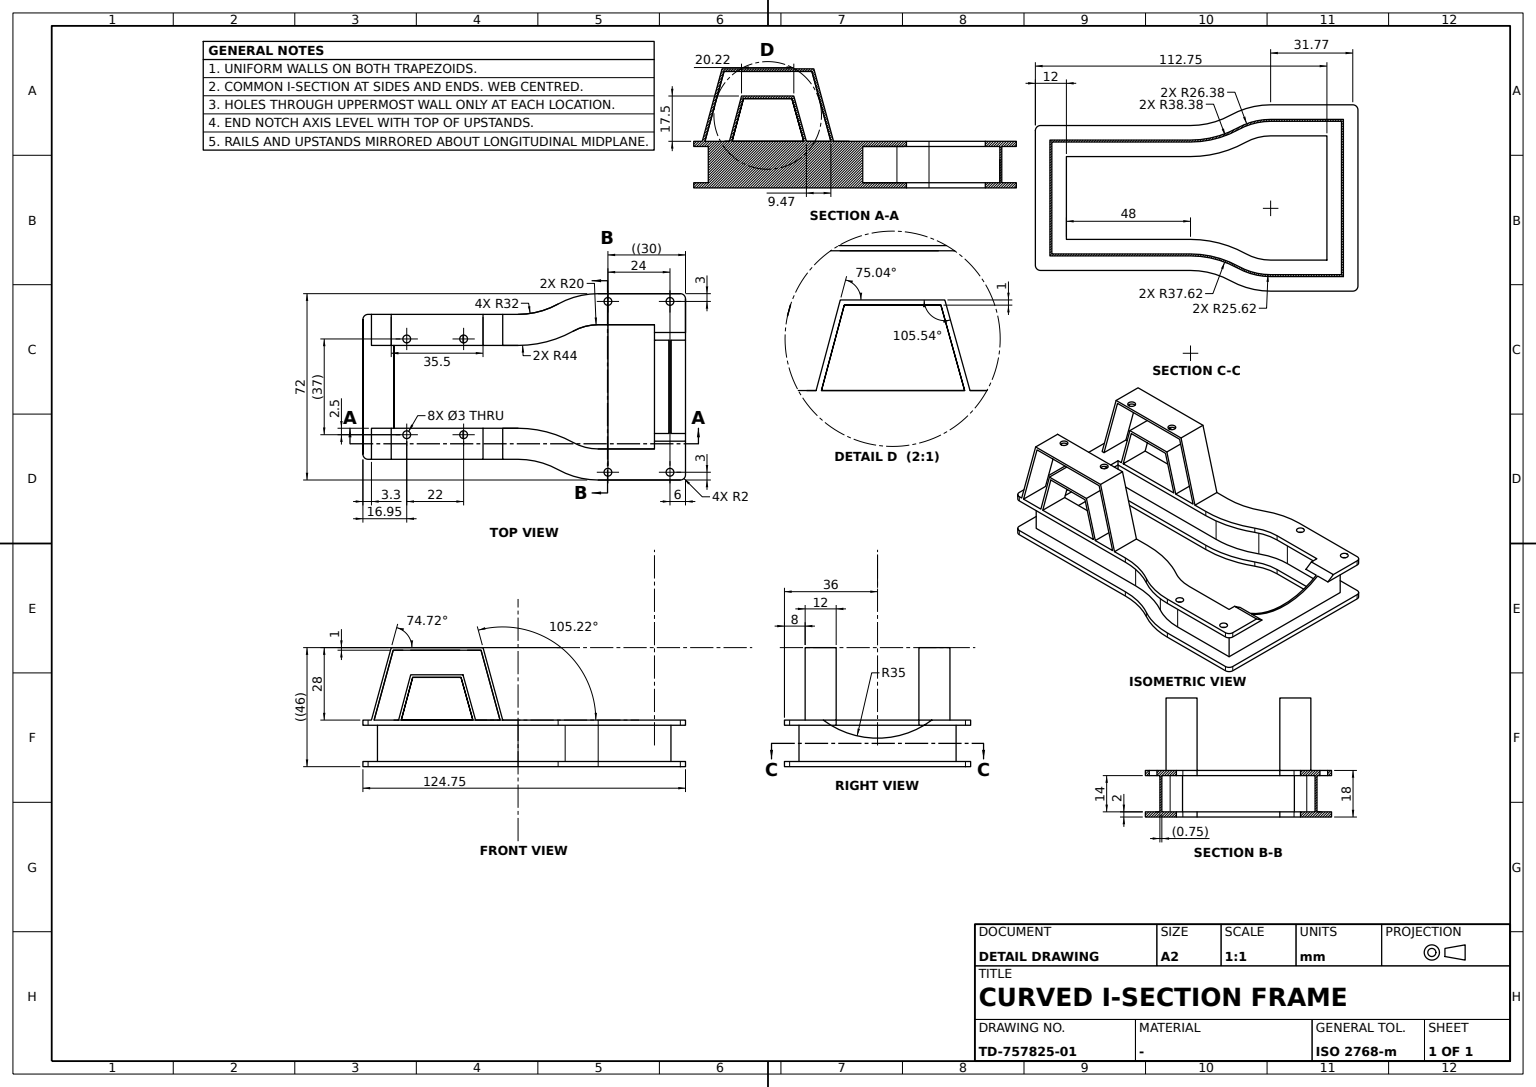
solid
v1 (-27.078125,72.215125,7)
v2 (-30.375,84.983867,7)
e1 v1 v2 CIRCLE(AX(P(-4,84.983867,7),D(0,0,1),D(1,0,0)),26.375) rev
v3 (-30.375,84.983867,-7)
e2 v3 v2 LINE
v4 (-27.078125,72.215125,-7)
e3 v4 v3 CIRCLE(AX(P(-4,84.983867,-7),D(0,0,-1),D(-1,0,0)),26.375)
e4 v4 v1 LINE
face CYL(AX(P(-4,84.983867,0),D(0,0,-1),D(-0.875,-0.484122918,0)),26.375) [e1 -e2 -e3 e4]
v5 (-16,47.031009,9)
v6 (-16,37.565009,9)
e5 v5 v6 LINE
v7 (-28,47.031009,9)
e6 v7 v5 LINE
v8 (-28,37.565009,9)
e7 v8 v7 LINE
e8 v8 v6 LINE
face PLANE(AX(P(0,-6,9),D(0,0,-1),D(0,1,0))) rev [-e5 -e6 -e7 e8]
v9 (-28,36.527057,9)
v10 (-16,36.527057,9)
e9 v9 v10 LINE
v11 (-28,8.837722,9)
e10 v11 v9 LINE
v12 (-16,8.837722,9)
e11 v11 v12 LINE
e12 v10 v12 LINE
face PLANE(AX(P(0,-6,9),D(0,0,-1),D(0,1,0))) rev [-e9 -e10 e11 -e12]
v13 (-32,69.491933,-9)
v14 (-36,84.983867,-9)
e13 v13 v14 CIRCLE(AX(P(-4,84.983867,-9),D(0,0,1),D(1,0,0)),32) rev
v15 (-32,69.491933,-7)
e14 v13 v15 LINE
v16 (-36,84.983867,-7)
e15 v15 v16 CIRCLE(AX(P(-4,84.983867,-7),D(0,0,-1),D(-1,0,0)),32)
e16 v14 v16 LINE
face CYL(AX(P(-4,84.983867,0),D(0,0,-1),D(-0.875,-0.484122918,0)),32) [-e13 e14 e15 -e16]
v17 (20,32.949611,36)
e17 v17 v17 CIRCLE(AX(P(18.5,32.949611,36),D(0,0,1),D(1,0,0)),1.5)
v18 (20,32.949611,37)
e18 v18 v18 CIRCLE(AX(P(18.5,32.949611,37),D(0,0,1),D(1,0,0)),1.5)
face CYL(AX(P(18.5,32.949611,13.34),D(0,0,1),D(0,1,0)),1.5) rev [-e17] [e18]
v19 (-16,32.698119,26.5)
e19 v19 v6 LINE
v20 (-28,32.698119,26.5)
e20 v20 v8 LINE
e21 v20 v19 LINE
face PLANE(AX(P(28,32.698119,26.5),D(0,0.963435821,0.267939209),D(0,0.267939209,-0.963435821))) [e19 -e8 -e20 e21]
v21 (24,106.75,-7)
v22 (-24,106.75,-7)
e22 v21 v22 LINE
v23 (-24,106.75,-9)
e23 v23 v22 LINE
v24 (24,106.75,-9)
e24 v24 v23 LINE
e25 v24 v21 LINE
face PLANE(AX(P(42,106.75,-7),D(0,1,0),D(0,0,-1))) rev [e22 -e23 -e24 e25]
v25 (16,13.246024,25.5)
v26 (16,31.938275,25.5)
e26 v25 v26 LINE
v27 (16,8.837722,9)
e27 v27 v25 LINE
v28 (16,36.527057,9)
e28 v28 v27 LINE
e29 v26 v28 LINE
v29 (16,32.698119,26.5)
v30 (16,37.565009,9)
e30 v29 v30 LINE
v31 (16,47.031009,9)
e31 v31 v30 LINE
v32 (16,39.685325,36)
e32 v32 v31 LINE
v33 (16,5.713058,36)
e33 v33 v32 LINE
v34 (16,-1.663352,9)
e34 v34 v33 LINE
v35 (16,-2.7,9)
e35 v35 v34 LINE
v36 (16,4.949611,37)
e36 v35 v36 LINE
v37 (16,40.449611,37)
e37 v36 v37 LINE
v38 (16,48.067357,9)
e38 v37 v38 LINE
v39 (16,54,9)
e39 v39 v38 LINE
v40 (16,54,7)
e40 v39 v40 LINE
v41 (16,6,7)
e41 v41 v40 LINE
v42 (16,6,9)
e42 v41 v42 LINE
v43 (16,7.802648,9)
e43 v43 v42 LINE
v44 (16,12.478119,26.5)
e44 v43 v44 LINE
e45 v44 v29 LINE
face PLANE(AX(P(16,-12,-7),D(1,0,0),D(0,0,-1))) rev [-e26 -e27 -e28 -e29] [e30 -e31 -e32 -e33 -e34 -e35 e36 e37 e38 -e39 e40 -e41 e42 -e43 e44 e45]
v45 (24,84.983867,-7)
v46 (24,84.983867,-9)
e46 v45 v46 LINE
e47 v45 v21 LINE
e48 v46 v24 LINE
face PLANE(AX(P(24,84.983867,-7),D(1,0,0),D(0,0,-1))) rev [-e46 e47 -e25 -e48]
v47 (28,-1.663352,9)
e49 v47 v34 LINE
v48 (28,5.713058,36)
e50 v48 v33 LINE
e51 v47 v48 LINE
face PLANE(AX(P(28,-1.663352,9),D(0,-0.964647876,0.263542168),D(0,0.263542168,0.964647876))) rev [e49 e34 -e50 -e51]
v49 (24,84.983867,9)
v50 (24,84.983867,7)
e52 v49 v50 LINE
v51 (21.5,75.301408,7)
e53 v51 v50 CIRCLE(AX(P(4,84.983867,7),D(0,0,1),D(1,0,0)),20)
v52 (21.5,75.301408,9)
e54 v52 v51 LINE
e55 v52 v49 CIRCLE(AX(P(4,84.983867,9),D(0,0,-1),D(-1,0,0)),20) rev
face CYL(AX(P(4,84.983867,0),D(0,0,1),D(0.875,-0.484122918,0)),20) rev [e52 -e53 -e54 e55]
v53 (-29.625,84.983867,7)
v54 (-29.625,112.375,7)
e56 v53 v54 LINE
v55 (-29.625,84.983867,-7)
e57 v53 v55 LINE
v56 (-29.625,112.375,-7)
e58 v55 v56 LINE
e59 v56 v54 LINE
face PLANE(AX(P(-29.625,84.983867,7),D(1,0,0),D(0,0,-1))) [-e56 e57 e58 e59]
v57 (22.375,54,-7)
v58 (22.375,54,7)
e60 v57 v58 LINE
v59 (22.375,-0.375,7)
e61 v59 v58 LINE
v60 (22.375,-0.375,-7)
e62 v59 v60 LINE
e63 v60 v57 LINE
face PLANE(AX(P(22.375,-12,-7),D(-1,0,0),D(0,0,1))) rev [e60 -e61 e62 e63]
v61 (31.5,88.75,9)
e64 v61 v61 CIRCLE(AX(P(33,88.75,9),D(0,0,-1),D(-1,0,0)),1.5) rev
v62 (34.5,88.75,7)
e65 v62 v62 CIRCLE(AX(P(33,88.75,7),D(0,0,1),D(1,0,0)),1.5)
face CYL(AX(P(33,88.75,-0.66),D(0,0,1),D(0,1,0)),1.5) rev [e64] [-e65]
v63 (-28,12.478119,26.5)
e66 v63 v20 LINE
v64 (-16,12.478119,26.5)
e67 v63 v64 LINE
e68 v64 v19 LINE
face PLANE(AX(P(28,12.478119,26.5),D(0,0,1),D(0,1,0))) [-e66 e67 e68 -e21]
v65 (32,69.491933,7)
v66 (32,69.491933,9)
e69 v65 v66 LINE
v67 (36,84.983867,7)
e70 v65 v67 CIRCLE(AX(P(4,84.983867,7),D(0,0,1),D(1,0,0)),32)
v68 (36,84.983867,9)
e71 v67 v68 LINE
e72 v66 v68 CIRCLE(AX(P(4,84.983867,9),D(0,0,-1),D(-1,0,0)),32) rev
face CYL(AX(P(4,84.983867,0),D(0,0,1),D(0.875,-0.484122918,0)),32) [-e69 e70 e71 -e72]
v69 (-26,-6,7)
v70 (26,-6,7)
e73 v69 v70 LINE
v71 (26,-6,9)
e74 v70 v71 LINE
v72 (-26,-6,9)
e75 v72 v71 LINE
e76 v69 v72 LINE
face PLANE(AX(P(0,-6,-9),D(0,1,0),D(0,0,1))) rev [e73 e74 -e75 -e76]
v73 (28,-4,7)
v74 (28,-4,9)
e77 v73 v74 LINE
e78 v74 v71 CIRCLE(AX(P(26,-4,9),D(0,0,-1),D(-1,0,0)),2)
e79 v70 v73 CIRCLE(AX(P(26,-4,7),D(0,0,1),D(1,0,0)),2)
face CYL(AX(P(26,-4,22),D(0,0,1),D(1,0,0)),2) [e77 e78 -e74 e79]
v75 (-16,6,-9)
v76 (-16,54,-9)
e80 v75 v76 LINE
v77 (-16,54,-7)
e81 v77 v76 LINE
v78 (-16,6,-7)
e82 v78 v77 LINE
e83 v75 v78 LINE
face PLANE(AX(P(-16,-12,-7),D(1,0,0),D(0,0,-1))) [e80 -e81 -e82 -e83]
v79 (34,118.75,7)
v80 (34,118.75,9)
e84 v79 v80 LINE
v81 (18.027756,118.75,7)
e85 v79 v81 LINE
v82 (21,118.75,9)
e86 v81 v82 CIRCLE(AX(P(0,118.75,37),D(0,-1,0),D(0,0,-1)),35)
e87 v80 v82 LINE
face PLANE(AX(P(42,118.75,-9),D(0,-1,0),D(0,0,1))) rev [-e84 e85 e86 -e87]
v83 (-31.5,88.75,7)
e88 v83 v83 CIRCLE(AX(P(-33,88.75,7),D(0,0,1),D(1,0,0)),1.5)
v84 (-34.5,88.75,9)
e89 v84 v84 CIRCLE(AX(P(-33,88.75,9),D(0,0,-1),D(-1,0,0)),1.5) rev
face CYL(AX(P(-33,88.75,-0.66),D(0,0,1),D(0,1,0)),1.5) rev [-e88] [e89]
v85 (-28,-2.7,9)
v86 (-16,-2.7,9)
e90 v85 v86 LINE
v87 (-16,4.949611,37)
e91 v86 v87 LINE
v88 (-28,4.949611,37)
e92 v88 v87 LINE
e93 v85 v88 LINE
face PLANE(AX(P(28,-2.7,9),D(0,-0.964647876,0.263542168),D(0,0.263542168,0.964647876))) [e90 e91 -e92 -e93]
v89 (36,116.75,9)
e94 v68 v89 LINE
v90 (36,116.75,7)
e95 v67 v90 LINE
e96 v90 v89 LINE
face PLANE(AX(P(36,84.983867,-9),D(-1,0,0),D(0,0,1))) rev [-e94 -e71 e95 e96]
v91 (-28,-4,7)
e97 v91 v69 CIRCLE(AX(P(-26,-4,7),D(0,0,1),D(1,0,0)),2)
v92 (-28,-4,9)
e98 v72 v92 CIRCLE(AX(P(-26,-4,9),D(0,0,-1),D(-1,0,0)),2)
e99 v91 v92 LINE
face CYL(AX(P(-26,-4,22),D(0,0,1),D(0,-1,0)),2) [e97 e76 e98 -e99]
v93 (28,4.949611,37)
e100 v93 v36 LINE
v94 (28,40.449611,37)
e101 v93 v94 LINE
e102 v94 v37 LINE
v95 (20,10.949611,37)
e103 v95 v95 CIRCLE(AX(P(18.5,10.949611,37),D(0,0,1),D(1,0,0)),1.5)
face PLANE(AX(P(28,4.949611,37),D(0,0,1),D(0,1,0))) [-e18] [-e37 -e100 e101 e102] [-e103]
v96 (18.027756,113.125,7)
e104 v96 v81 LINE
v97 (-18.027756,113.125,7)
e105 v97 v96 CIRCLE(AX(P(0,113.125,37),D(0,-1,0),D(0,0,-1)),35)
v98 (-18.027756,118.75,7)
e106 v98 v97 LINE
v99 (-21,118.75,9)
e107 v99 v98 CIRCLE(AX(P(0,118.75,37),D(0,-1,0),D(0,0,-1)),35)
v100 (-21,106.75,9)
e108 v100 v99 LINE
v101 (-18.027756,106.75,7)
e109 v101 v100 CIRCLE(AX(P(0,106.75,37),D(0,1,0),D(0,0,1)),35)
v102 (-18.027756,112.375,7)
e110 v102 v101 LINE
v103 (18.027756,112.375,7)
e111 v103 v102 CIRCLE(AX(P(0,112.375,37),D(0,1,0),D(0,0,1)),35)
v104 (18.027756,106.75,7)
e112 v104 v103 LINE
v105 (21,106.75,9)
e113 v105 v104 CIRCLE(AX(P(0,106.75,37),D(0,1,0),D(0,0,1)),35)
e114 v82 v105 LINE
face CYL(AX(P(0,115.75,37),D(0,1,0),D(-1,0,0)),35) rev [-e104 -e105 -e106 -e107 -e108 -e109 -e110 -e111 -e112 -e113 -e114 -e86]
v106 (-17,10.949611,36)
e115 v106 v106 CIRCLE(AX(P(-18.5,10.949611,36),D(0,0,1),D(1,0,0)),1.5)
v107 (-17,10.949611,37)
e116 v107 v107 CIRCLE(AX(P(-18.5,10.949611,37),D(0,0,1),D(1,0,0)),1.5)
face CYL(AX(P(-18.5,10.949611,13.34),D(0,0,1),D(0,1,0)),1.5) rev [-e115] [e116]
v108 (-28,54,7)
e117 v91 v108 LINE
v109 (-32,69.491933,7)
e118 v109 v108 CIRCLE(AX(P(-60,54,7),D(0,0,1),D(1,0,0)),32) rev
v110 (-36,84.983867,7)
e119 v109 v110 CIRCLE(AX(P(-4,84.983867,7),D(0,0,1),D(1,0,0)),32) rev
v111 (-36,116.75,7)
e120 v110 v111 LINE
v112 (-34,118.75,7)
e121 v112 v111 CIRCLE(AX(P(-34,116.75,7),D(0,0,1),D(1,0,0)),2)
e122 v98 v112 LINE
v113 (-30.375,113.125,7)
e123 v97 v113 LINE
e124 v2 v113 LINE
v114 (-22.375,54,7)
e125 v1 v114 CIRCLE(AX(P(-60,54,7),D(0,0,1),D(1,0,0)),37.625) rev
v115 (-22.375,-0.375,7)
e126 v115 v114 LINE
e127 v115 v59 LINE
v116 (27.078125,72.215125,7)
e128 v116 v58 CIRCLE(AX(P(60,54,7),D(0,0,1),D(1,0,0)),37.625)
v117 (30.375,84.983867,7)
e129 v116 v117 CIRCLE(AX(P(4,84.983867,7),D(0,0,1),D(1,0,0)),26.375)
v118 (30.375,113.125,7)
e130 v117 v118 LINE
e131 v118 v96 LINE
e132 v90 v79 CIRCLE(AX(P(34,116.75,7),D(0,0,1),D(1,0,0)),2)
v119 (28,54,7)
e133 v65 v119 CIRCLE(AX(P(60,54,7),D(0,0,1),D(1,0,0)),32)
e134 v73 v119 LINE
v120 (-31.5,112.75,7)
e135 v120 v120 CIRCLE(AX(P(-33,112.75,7),D(0,0,1),D(1,0,0)),1.5)
v121 (34.5,112.75,7)
e136 v121 v121 CIRCLE(AX(P(33,112.75,7),D(0,0,1),D(1,0,0)),1.5)
face PLANE(AX(P(0,6,7),D(0,0,1),D(0,-1,0))) rev [e88] [-e97 e117 -e118 e119 e120 -e121 -e122 e106 e123 -e124 -e1 e125 -e126 e127 e61 -e128 e129 e130 e131 e104 -e85 -e132 -e95 -e70 e133 -e134 -e79 -e73] [e65] [e135] [e136]
v122 (16,54,-7)
v123 (16,54,-9)
e137 v122 v123 LINE
v124 (21.5,75.301408,-7)
e138 v124 v122 CIRCLE(AX(P(60,54,-7),D(0,0,-1),D(-1,0,0)),44) rev
v125 (21.5,75.301408,-9)
e139 v124 v125 LINE
e140 v125 v123 CIRCLE(AX(P(60,54,-9),D(0,0,1),D(1,0,0)),44)
face CYL(AX(P(60,54,0),D(0,0,1),D(-0.875,0.484122918,0)),44) [-e137 -e138 e139 e140]
e141 v125 v46 CIRCLE(AX(P(4,84.983867,-9),D(0,0,1),D(1,0,0)),20)
e142 v124 v45 CIRCLE(AX(P(4,84.983867,-7),D(0,0,-1),D(-1,0,0)),20) rev
face CYL(AX(P(4,84.983867,0),D(0,0,1),D(0.875,-0.484122918,0)),20) rev [e46 -e141 -e139 e142]
v126 (-21.5,75.301408,-7)
v127 (-24,84.983867,-7)
e143 v126 v127 CIRCLE(AX(P(-4,84.983867,-7),D(0,0,-1),D(-1,0,0)),20)
v128 (-21.5,75.301408,-9)
e144 v126 v128 LINE
v129 (-24,84.983867,-9)
e145 v128 v129 CIRCLE(AX(P(-4,84.983867,-9),D(0,0,1),D(1,0,0)),20) rev
e146 v127 v129 LINE
face CYL(AX(P(-4,84.983867,0),D(0,0,-1),D(-0.875,-0.484122918,0)),20) rev [-e143 e144 e145 -e146]
v130 (28,7.802648,9)
e147 v130 v43 LINE
v131 (28,12.478119,26.5)
e148 v130 v131 LINE
e149 v131 v44 LINE
face PLANE(AX(P(28,7.802648,9),D(0,-0.966113825,0.258116404),D(0,0.258116404,0.966113825))) [-e147 e148 e149 -e44]
v132 (28,8.837722,9)
e150 v132 v27 LINE
v133 (28,13.246024,25.5)
e151 v133 v25 LINE
e152 v132 v133 LINE
face PLANE(AX(P(28,8.837722,9),D(0,-0.966113825,0.258116404),D(0,0.258116404,0.966113825))) rev [e150 e27 -e151 -e152]
v134 (-28,39.685325,36)
e153 v134 v7 LINE
v135 (-16,39.685325,36)
e154 v135 v5 LINE
e155 v134 v135 LINE
face PLANE(AX(P(28,39.685325,36),D(0,0.964926501,0.262520187),D(0,0.262520187,-0.964926501))) rev [e153 e6 -e154 -e155]
v136 (-22.375,-0.375,-7)
v137 (-22.375,54,-7)
e156 v136 v137 LINE
e157 v115 v136 LINE
e158 v137 v114 LINE
face PLANE(AX(P(-22.375,-12,-7),D(-1,0,0),D(0,0,1))) [-e156 -e157 e126 -e158]
v138 (-16,6,7)
e159 v138 v41 LINE
v139 (-16,6,9)
e160 v138 v139 LINE
e161 v139 v42 LINE
face PLANE(AX(P(0,6,-7),D(0,-1,0),D(0,0,-1))) rev [-e159 e160 e161 -e42]
v140 (21.625,54,7)
v141 (21.625,54,-7)
e162 v140 v141 LINE
v142 (26.421875,72.578217,7)
e163 v142 v140 CIRCLE(AX(P(60,54,7),D(0,0,1),D(1,0,0)),38.375)
v143 (26.421875,72.578217,-7)
e164 v142 v143 LINE
e165 v143 v141 CIRCLE(AX(P(60,54,-7),D(0,0,-1),D(-1,0,0)),38.375) rev
face CYL(AX(P(60,54,0),D(0,0,1),D(-0.875,0.484122918,0)),38.375) [-e162 -e163 e164 e165]
v144 (20,10.949611,36)
e166 v144 v144 CIRCLE(AX(P(18.5,10.949611,36),D(0,0,1),D(1,0,0)),1.5)
v145 (28,39.685325,36)
e167 v145 v32 LINE
e168 v48 v145 LINE
face PLANE(AX(P(28,5.713058,36),D(0,0,1),D(0,1,0))) rev [e17] [e166] [e50 e33 -e167 -e168]
v146 (-32,69.491933,9)
e169 v109 v146 LINE
v147 (-36,84.983867,9)
e170 v146 v147 CIRCLE(AX(P(-4,84.983867,9),D(0,0,-1),D(-1,0,0)),32)
e171 v110 v147 LINE
face CYL(AX(P(-4,84.983867,0),D(0,0,-1),D(-0.875,-0.484122918,0)),32) [-e119 e169 e170 -e171]
v148 (28,36.527057,9)
e172 v132 v148 LINE
e173 v148 v28 LINE
face PLANE(AX(P(0,-6,9),D(0,0,-1),D(0,1,0))) rev [e28 -e150 e172 e173]
v149 (28,32.698119,26.5)
e174 v149 v29 LINE
v150 (28,37.565009,9)
e175 v149 v150 LINE
e176 v150 v30 LINE
face PLANE(AX(P(28,32.698119,26.5),D(0,0.963435821,0.267939209),D(0,0.267939209,-0.963435821))) [-e174 e175 e176 -e30]
v151 (-21.625,0.375,-7)
v152 (-21.625,0.375,7)
e177 v151 v152 LINE
v153 (21.625,0.375,7)
e178 v152 v153 LINE
v154 (21.625,0.375,-7)
e179 v154 v153 LINE
e180 v151 v154 LINE
face PLANE(AX(P(0,0.375,7),D(0,-1,0),D(0,0,-1))) rev [e177 e178 -e179 -e180]
e181 v129 v23 LINE
e182 v127 v22 LINE
face PLANE(AX(P(-24,84.983867,-7),D(1,0,0),D(0,0,-1))) [e146 e181 e23 -e182]
v155 (-24,84.983867,9)
v156 (-24,106.75,9)
e183 v155 v156 LINE
v157 (-24,84.983867,7)
e184 v155 v157 LINE
v158 (-24,106.75,7)
e185 v157 v158 LINE
e186 v158 v156 LINE
face PLANE(AX(P(-24,84.983867,-7),D(1,0,0),D(0,0,-1))) [-e183 e184 e185 e186]
e187 v126 v77 CIRCLE(AX(P(-60,54,-7),D(0,0,-1),D(-1,0,0)),44)
v159 (16,6,-7)
e188 v159 v122 LINE
e189 v78 v159 LINE
v160 (-26.421875,72.578217,-7)
v161 (-21.625,54,-7)
e190 v160 v161 CIRCLE(AX(P(-60,54,-7),D(0,0,-1),D(-1,0,0)),38.375)
e191 v151 v161 LINE
e192 v154 v141 LINE
v162 (29.625,84.983867,-7)
e193 v143 v162 CIRCLE(AX(P(4,84.983867,-7),D(0,0,-1),D(-1,0,0)),25.625) rev
v163 (29.625,112.375,-7)
e194 v162 v163 LINE
e195 v163 v56 LINE
e196 v160 v55 CIRCLE(AX(P(-4,84.983867,-7),D(0,0,-1),D(-1,0,0)),25.625)
face PLANE(AX(P(0,-6,-7),D(0,0,-1),D(0,1,0))) rev [-e187 e143 e182 -e22 -e47 -e142 e138 -e188 -e189 e82] [e190 -e191 e180 e192 -e165 e193 e194 e195 -e58 -e196]
v164 (28,47.031009,9)
e197 v150 v164 LINE
e198 v164 v31 LINE
face PLANE(AX(P(0,-6,9),D(0,0,-1),D(0,1,0))) rev [e31 -e176 e197 e198]
v165 (31.5,112.75,9)
e199 v165 v165 CIRCLE(AX(P(33,112.75,9),D(0,0,-1),D(-1,0,0)),1.5) rev
v166 (28,48.067357,9)
e200 v166 v38 LINE
v167 (28,54,9)
e201 v166 v167 LINE
e202 v66 v167 CIRCLE(AX(P(60,54,9),D(0,0,-1),D(-1,0,0)),32) rev
e203 v80 v89 CIRCLE(AX(P(34,116.75,9),D(0,0,-1),D(-1,0,0)),2)
v168 (24,106.75,9)
e204 v168 v105 LINE
e205 v49 v168 LINE
e206 v52 v39 CIRCLE(AX(P(60,54,9),D(0,0,-1),D(-1,0,0)),44) rev
face PLANE(AX(P(0,-6,9),D(0,0,-1),D(0,1,0))) rev [-e199] [-e200 e201 -e202 e72 e94 -e203 e87 e114 -e204 -e205 -e55 e206 e39] [-e64]
v169 (27.078125,72.215125,-7)
e207 v169 v116 LINE
v170 (30.375,84.983867,-7)
e208 v169 v170 CIRCLE(AX(P(4,84.983867,-7),D(0,0,-1),D(-1,0,0)),26.375) rev
e209 v170 v117 LINE
face CYL(AX(P(4,84.983867,0),D(0,0,1),D(0.875,-0.484122918,0)),26.375) [-e207 e208 e209 -e129]
v171 (-28,48.067357,9)
v172 (-16,48.067357,9)
e210 v171 v172 LINE
v173 (-16,54,9)
e211 v173 v172 LINE
v174 (-21.5,75.301408,9)
e212 v174 v173 CIRCLE(AX(P(-60,54,9),D(0,0,-1),D(-1,0,0)),44)
e213 v174 v155 CIRCLE(AX(P(-4,84.983867,9),D(0,0,-1),D(-1,0,0)),20)
e214 v100 v156 LINE
v175 (-34,118.75,9)
e215 v99 v175 LINE
v176 (-36,116.75,9)
e216 v176 v175 CIRCLE(AX(P(-34,116.75,9),D(0,0,-1),D(-1,0,0)),2)
e217 v147 v176 LINE
v177 (-28,54,9)
e218 v146 v177 CIRCLE(AX(P(-60,54,9),D(0,0,-1),D(-1,0,0)),32)
e219 v171 v177 LINE
v178 (-34.5,112.75,9)
e220 v178 v178 CIRCLE(AX(P(-33,112.75,9),D(0,0,-1),D(-1,0,0)),1.5) rev
face PLANE(AX(P(0,-6,9),D(0,0,-1),D(0,1,0))) rev [e210 -e211 -e212 e213 e183 -e214 e108 e215 -e216 -e217 -e170 e218 -e219] [-e89] [-e220]
e221 v145 v164 LINE
face PLANE(AX(P(28,39.685325,36),D(0,0.964926501,0.262520187),D(0,0.262520187,-0.964926501))) rev [-e221 e167 e32 -e198]
v179 (28,31.938275,25.5)
e222 v179 v26 LINE
e223 v133 v179 LINE
face PLANE(AX(P(28,13.246024,25.5),D(0,0,1),D(0,1,0))) rev [-e222 -e223 e151 e26]
v180 (34,118.75,-9)
v181 (-34,118.75,-9)
e224 v180 v181 LINE
v182 (-34,118.75,-7)
e225 v181 v182 LINE
v183 (34,118.75,-7)
e226 v183 v182 LINE
e227 v180 v183 LINE
face PLANE(AX(P(42,118.75,-9),D(0,-1,0),D(0,0,1))) rev [e224 e225 -e226 -e227]
e228 v119 v167 LINE
face CYL(AX(P(60,54,0),D(0,0,1),D(-0.875,0.484122918,0)),32) rev [e69 e202 -e228 -e133]
e229 v131 v149 LINE
face PLANE(AX(P(28,12.478119,26.5),D(0,0,1),D(0,1,0))) [-e45 -e149 e229 e174]
v184 (28,54,-9)
v185 (28,54,-7)
e230 v184 v185 LINE
v186 (32,69.491933,-9)
e231 v186 v184 CIRCLE(AX(P(60,54,-9),D(0,0,1),D(1,0,0)),32)
v187 (32,69.491933,-7)
e232 v186 v187 LINE
e233 v187 v185 CIRCLE(AX(P(60,54,-7),D(0,0,-1),D(-1,0,0)),32) rev
face CYL(AX(P(60,54,0),D(0,0,1),D(-0.875,0.484122918,0)),32) rev [-e230 -e231 e232 e233]
face CYL(AX(P(34,116.75,8),D(0,0,1),D(0,1,0)),2) [e203 -e96 e132 e84]
v188 (-21.5,75.301408,7)
v189 (-16,54,7)
e234 v188 v189 CIRCLE(AX(P(-60,54,7),D(0,0,1),D(1,0,0)),44) rev
e235 v174 v188 LINE
e236 v173 v189 LINE
face CYL(AX(P(-60,54,0),D(0,0,-1),D(0.875,0.484122918,0)),44) [-e234 -e235 e212 e236]
v190 (-28,-4,-9)
v191 (-28,-4,-7)
e237 v190 v191 LINE
v192 (-28,54,-7)
e238 v191 v192 LINE
v193 (-28,54,-9)
e239 v193 v192 LINE
e240 v190 v193 LINE
face PLANE(AX(P(-28,-12,-9),D(-1,0,0),D(0,0,1))) [e237 e238 -e239 -e240]
v194 (-28,7.802648,9)
e241 v194 v63 LINE
v195 (-28,5.713058,36)
e242 v195 v134 LINE
v196 (-28,-1.663352,9)
e243 v196 v195 LINE
e244 v196 v194 LINE
e245 v92 v85 LINE
v197 (-28,40.449611,37)
e246 v88 v197 LINE
e247 v197 v171 LINE
e248 v108 v177 LINE
v198 (-28,13.246024,25.5)
v199 (-28,31.938275,25.5)
e249 v198 v199 LINE
e250 v11 v198 LINE
e251 v199 v9 LINE
face PLANE(AX(P(-28,-12,-9),D(-1,0,0),D(0,0,1))) [e241 e66 e20 e7 -e153 -e242 -e243 e244] [-e117 e99 e245 e93 e246 e247 e219 -e248] [-e249 -e250 e10 -e251]
e252 v128 v76 CIRCLE(AX(P(-60,54,-9),D(0,0,1),D(1,0,0)),44) rev
face CYL(AX(P(-60,54,0),D(0,0,-1),D(0.875,0.484122918,0)),44) [e81 -e252 -e144 e187]
v200 (-30.375,113.125,-7)
e253 v113 v200 LINE
e254 v3 v200 LINE
face PLANE(AX(P(-30.375,84.983867,-7),D(-1,0,0),D(0,0,1))) [e2 e124 e253 -e254]
v201 (-16,40.449611,37)
e255 v197 v201 LINE
e256 v201 v172 LINE
face PLANE(AX(P(28,40.449611,37),D(0,0.964926501,0.262520187),D(0,0.262520187,-0.964926501))) [-e210 -e247 e255 e256]
v202 (24,106.75,7)
e257 v202 v168 LINE
e258 v202 v104 LINE
face PLANE(AX(P(42,106.75,-7),D(0,1,0),D(0,0,-1))) rev [e257 e204 e113 -e258]
e259 v111 v176 LINE
face PLANE(AX(P(-36,84.983867,-9),D(-1,0,0),D(0,0,1))) [-e120 e171 e217 -e259]
face CYL(AX(P(33,112.75,-0.66),D(0,0,1),D(0,1,0)),1.5) rev [-e136] [e199]
v203 (28,-4,-9)
v204 (28,-4,-7)
e260 v203 v204 LINE
v205 (26,-6,-7)
e261 v204 v205 CIRCLE(AX(P(26,-4,-7),D(0,0,-1),D(-1,0,0)),2)
v206 (26,-6,-9)
e262 v206 v205 LINE
e263 v206 v203 CIRCLE(AX(P(26,-4,-9),D(0,0,1),D(1,0,0)),2)
face CYL(AX(P(26,-4,22),D(0,0,1),D(1,0,0)),2) [e260 e261 -e262 e263]
v207 (-16,13.246024,25.5)
v208 (-16,31.938275,25.5)
e264 v207 v208 LINE
e265 v198 v207 LINE
e266 v199 v208 LINE
face PLANE(AX(P(28,13.246024,25.5),D(0,0,1),D(0,1,0))) rev [-e264 -e265 e249 e266]
v209 (-26.421875,72.578217,7)
e267 v209 v160 LINE
e268 v209 v53 CIRCLE(AX(P(-4,84.983867,7),D(0,0,1),D(1,0,0)),25.625) rev
face CYL(AX(P(-4,84.983867,0),D(0,0,-1),D(-0.875,-0.484122918,0)),25.625) rev [e267 e196 -e57 -e268]
e269 v203 v184 LINE
e270 v204 v185 LINE
face PLANE(AX(P(28,-12,-9),D(-1,0,0),D(0,0,1))) rev [e269 e230 -e270 -e260]
v210 (-21.625,54,7)
e271 v210 v161 LINE
e272 v152 v210 LINE
face PLANE(AX(P(-21.625,-12,7),D(1,0,0),D(0,0,-1))) [-e177 e191 -e271 -e272]
e273 v94 v166 LINE
face PLANE(AX(P(28,40.449611,37),D(0,0.964926501,0.262520187),D(0,0.262520187,-0.964926501))) [-e38 -e102 e273 e200]
face CYL(AX(P(18.5,10.949611,13.34),D(0,0,1),D(0,1,0)),1.5) rev [-e166] [e103]
v211 (-36,116.75,-9)
e274 v14 v211 LINE
e275 v181 v211 CIRCLE(AX(P(-34,116.75,-9),D(0,0,1),D(1,0,0)),2)
v212 (36,116.75,-9)
e276 v212 v180 CIRCLE(AX(P(34,116.75,-9),D(0,0,1),D(1,0,0)),2)
v213 (36,84.983867,-9)
e277 v213 v212 LINE
e278 v186 v213 CIRCLE(AX(P(4,84.983867,-9),D(0,0,1),D(1,0,0)),32)
v214 (-26,-6,-9)
e279 v214 v206 LINE
e280 v190 v214 CIRCLE(AX(P(-26,-4,-9),D(0,0,1),D(1,0,0)),2)
e281 v13 v193 CIRCLE(AX(P(-60,54,-9),D(0,0,1),D(1,0,0)),32) rev
v215 (16,6,-9)
e282 v75 v215 LINE
e283 v215 v123 LINE
face PLANE(AX(P(0,6,-9),D(0,0,1),D(0,-1,0))) rev [e13 e274 -e275 -e224 -e276 -e277 -e278 e231 -e269 -e263 -e279 -e280 e240 -e281] [-e80 e282 e283 -e140 e141 e48 e24 -e181 -e145 e252]
e284 v112 v175 LINE
face CYL(AX(P(-34,116.75,8),D(0,0,1),D(-1,0,0)),2) [-e284 e121 e259 e216]
e285 v209 v210 CIRCLE(AX(P(-60,54,7),D(0,0,1),D(1,0,0)),38.375) rev
e286 v102 v54 LINE
e287 v101 v158 LINE
e288 v188 v157 CIRCLE(AX(P(-4,84.983867,7),D(0,0,1),D(1,0,0)),20) rev
e289 v138 v189 LINE
e290 v51 v40 CIRCLE(AX(P(60,54,7),D(0,0,1),D(1,0,0)),44)
e291 v50 v202 LINE
v216 (29.625,112.375,7)
e292 v216 v103 LINE
v217 (29.625,84.983867,7)
e293 v217 v216 LINE
e294 v142 v217 CIRCLE(AX(P(4,84.983867,7),D(0,0,1),D(1,0,0)),25.625)
e295 v153 v140 LINE
face PLANE(AX(P(0,6,7),D(0,0,1),D(0,-1,0))) rev [-e178 e272 -e285 e268 e56 -e286 e110 e287 -e185 -e288 e234 -e289 e159 e41 -e290 e53 e291 e258 e112 -e292 -e293 -e294 e163 -e295]
v218 (-36,116.75,-7)
e296 v218 v182 CIRCLE(AX(P(-34,116.75,-7),D(0,0,-1),D(-1,0,0)),2)
e297 v16 v218 LINE
e298 v15 v192 CIRCLE(AX(P(-60,54,-7),D(0,0,-1),D(-1,0,0)),32)
v219 (-26,-6,-7)
e299 v219 v191 CIRCLE(AX(P(-26,-4,-7),D(0,0,-1),D(-1,0,0)),2)
e300 v219 v205 LINE
v220 (36,84.983867,-7)
e301 v187 v220 CIRCLE(AX(P(4,84.983867,-7),D(0,0,-1),D(-1,0,0)),32) rev
v221 (36,116.75,-7)
e302 v220 v221 LINE
e303 v183 v221 CIRCLE(AX(P(34,116.75,-7),D(0,0,-1),D(-1,0,0)),2)
v222 (30.375,113.125,-7)
e304 v222 v200 LINE
e305 v170 v222 LINE
e306 v169 v57 CIRCLE(AX(P(60,54,-7),D(0,0,-1),D(-1,0,0)),37.625) rev
e307 v136 v60 LINE
e308 v4 v137 CIRCLE(AX(P(-60,54,-7),D(0,0,-1),D(-1,0,0)),37.625)
face PLANE(AX(P(0,-6,-7),D(0,0,-1),D(0,1,0))) rev [-e296 -e297 -e15 e298 -e238 -e299 e300 -e261 e270 -e233 e301 e302 -e303 e226] [e254 -e304 -e305 -e208 e306 -e63 -e307 e156 -e308 e3]
v223 (-16,7.802648,9)
e309 v223 v64 LINE
e310 v194 v223 LINE
face PLANE(AX(P(28,7.802648,9),D(0,-0.966113825,0.258116404),D(0,0.258116404,0.966113825))) [e309 -e67 -e241 e310]
face CYL(AX(P(-60,54,0),D(0,0,-1),D(0.875,0.484122918,0)),37.625) rev [-e125 -e4 e308 e158]
face CYL(AX(P(-60,54,0),D(0,0,-1),D(0.875,0.484122918,0)),32) rev [e239 -e298 -e14 e281]
e311 v211 v218 LINE
face CYL(AX(P(-34,116.75,8),D(0,0,1),D(-1,0,0)),2) [-e225 e275 e311 e296]
face CYL(AX(P(60,54,0),D(0,0,1),D(-0.875,0.484122918,0)),44) [e290 -e40 -e206 e54]
e312 v214 v219 LINE
face CYL(AX(P(-26,-4,22),D(0,0,1),D(0,-1,0)),2) [e312 e299 -e237 e280]
face PLANE(AX(P(21.625,-12,7),D(1,0,0),D(0,0,-1))) rev [e295 e162 -e192 e179]
e313 v87 v201 LINE
v224 (-17,32.949611,37)
e314 v224 v224 CIRCLE(AX(P(-18.5,32.949611,37),D(0,0,1),D(1,0,0)),1.5)
face PLANE(AX(P(28,4.949611,37),D(0,0,1),D(0,1,0))) [-e116] [e313 -e255 -e246 e92] [-e314]
e315 v212 v221 LINE
face CYL(AX(P(34,116.75,8),D(0,0,1),D(0,1,0)),2) [-e315 e276 e227 e303]
face PLANE(AX(P(42,118.75,-9),D(0,-1,0),D(0,0,1))) rev [e284 -e215 e107 e122]
face PLANE(AX(P(0,-0.375,-7),D(0,1,0),D(0,0,1))) rev [-e62 -e127 e157 e307]
face CYL(AX(P(-60,54,0),D(0,0,-1),D(0.875,0.484122918,0)),38.375) [-e190 -e267 e285 e271]
face PLANE(AX(P(0,-6,-9),D(0,1,0),D(0,0,1))) rev [-e312 e279 e262 -e300]
face PLANE(AX(P(-36,84.983867,-9),D(-1,0,0),D(0,0,1))) [-e311 -e274 e16 e297]
e316 v208 v10 LINE
face PLANE(AX(P(28,31.938275,25.5),D(0,0.963435821,0.267939209),D(0,0.267939209,-0.963435821))) rev [-e316 -e266 e251 e9]
e317 v217 v162 LINE
face CYL(AX(P(4,84.983867,0),D(0,0,1),D(0.875,-0.484122918,0)),25.625) rev [e317 -e193 -e164 e294]
e318 v118 v222 LINE
face PLANE(AX(P(42,113.125,-7),D(0,-1,0),D(0,0,1))) rev [-e253 -e123 e105 -e131 e318 e304]
face CYL(AX(P(60,54,0),D(0,0,1),D(-0.875,0.484122918,0)),37.625) rev [-e60 -e306 e207 e128]
v225 (28,-2.7,9)
e319 v225 v93 LINE
e320 v74 v225 LINE
e321 v47 v130 LINE
e322 v179 v148 LINE
face PLANE(AX(P(28,-12,-9),D(-1,0,0),D(0,0,1))) rev [-e273 -e101 -e319 -e320 -e77 e134 e228 -e201] [-e197 -e175 -e229 -e148 -e321 e51 e168 e221] [e322 -e172 e152 e223]
face PLANE(AX(P(28,31.938275,25.5),D(0,0.963435821,0.267939209),D(0,0.267939209,-0.963435821))) rev [e222 e29 -e173 -e322]
e323 v213 v220 LINE
face PLANE(AX(P(36,84.983867,-9),D(-1,0,0),D(0,0,1))) rev [e315 -e302 -e323 e277]
e324 v215 v159 LINE
face PLANE(AX(P(16,-12,-7),D(1,0,0),D(0,0,-1))) rev [-e283 e324 e188 e137]
face CYL(AX(P(-60,54,0),D(0,0,-1),D(0.875,0.484122918,0)),32) rev [-e218 -e169 e118 e248]
e325 v163 v216 LINE
face PLANE(AX(P(42,112.375,7),D(0,1,0),D(0,0,-1))) rev [e111 e286 -e59 -e195 e325 e292]
e326 v225 v35 LINE
e327 v223 v139 LINE
v226 (-16,-1.663352,9)
e328 v196 v226 LINE
e329 v86 v226 LINE
face PLANE(AX(P(0,-6,9),D(0,0,-1),D(0,1,0))) rev [-e245 -e98 e75 -e78 e320 e326 e35 -e49 e321 e147 e43 -e161 -e327 -e310 -e244 e328 -e329 -e90]
v227 (-17,32.949611,36)
e330 v227 v227 CIRCLE(AX(P(-18.5,32.949611,36),D(0,0,1),D(1,0,0)),1.5)
v228 (-16,5.713058,36)
e331 v228 v135 LINE
e332 v195 v228 LINE
face PLANE(AX(P(28,5.713058,36),D(0,0,1),D(0,1,0))) rev [e115] [e330] [e242 e155 -e331 -e332]
face PLANE(AX(P(24,84.983867,-7),D(1,0,0),D(0,0,-1))) rev [-e257 -e291 -e52 e205]
face CYL(AX(P(4,84.983867,0),D(0,0,1),D(0.875,-0.484122918,0)),32) [e323 -e301 -e232 e278]
face PLANE(AX(P(30.375,84.983867,-7),D(-1,0,0),D(0,0,1))) rev [e305 -e318 -e130 -e209]
e333 v226 v228 LINE
e334 v12 v207 LINE
face PLANE(AX(P(-16,-12,-7),D(1,0,0),D(0,0,-1))) [e331 e154 e5 -e19 -e68 -e309 e327 -e160 e289 -e236 e211 -e256 -e313 -e91 e329 e333] [e12 e334 e264 e316]
face PLANE(AX(P(28,-1.663352,9),D(0,-0.964647876,0.263542168),D(0,0.263542168,0.964647876))) rev [-e333 -e328 e243 e332]
face CYL(AX(P(-18.5,32.949611,13.34),D(0,0,1),D(0,1,0)),1.5) rev [e314] [-e330]
face PLANE(AX(P(42,106.75,-7),D(0,1,0),D(0,0,-1))) rev [e109 e214 -e186 -e287]
face CYL(AX(P(-4,84.983867,0),D(0,0,-1),D(-0.875,-0.484122918,0)),20) rev [-e213 e235 e288 -e184]
face PLANE(AX(P(29.625,84.983867,7),D(1,0,0),D(0,0,-1))) rev [-e194 -e317 e293 -e325]
face PLANE(AX(P(28,-2.7,9),D(0,-0.964647876,0.263542168),D(0,0.263542168,0.964647876))) [-e326 e319 e100 -e36]
face CYL(AX(P(-33,112.75,-0.66),D(0,0,1),D(0,1,0)),1.5) rev [-e135] [e220]
face PLANE(AX(P(0,6,-7),D(0,-1,0),D(0,0,-1))) rev [e189 -e324 -e282 e83]
face PLANE(AX(P(28,8.837722,9),D(0,-0.966113825,0.258116404),D(0,0.258116404,0.966113825))) rev [-e334 -e11 e250 e265]
